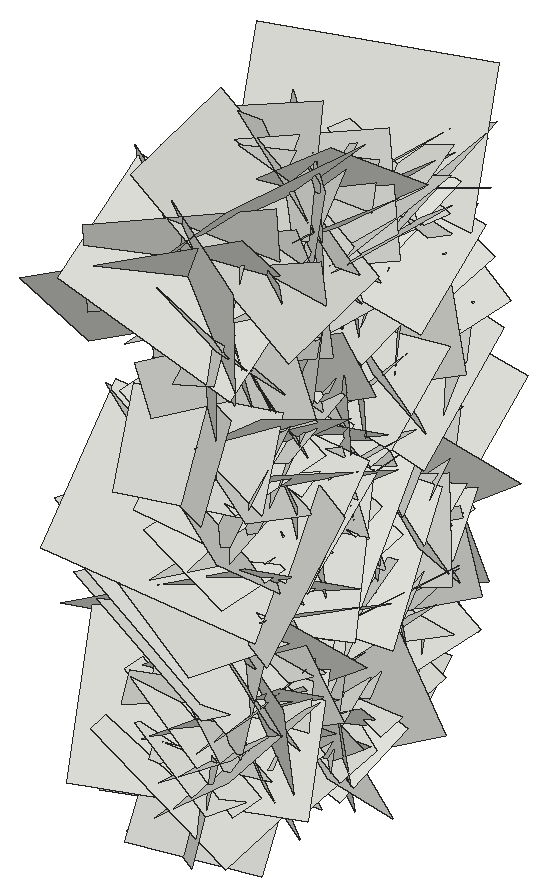
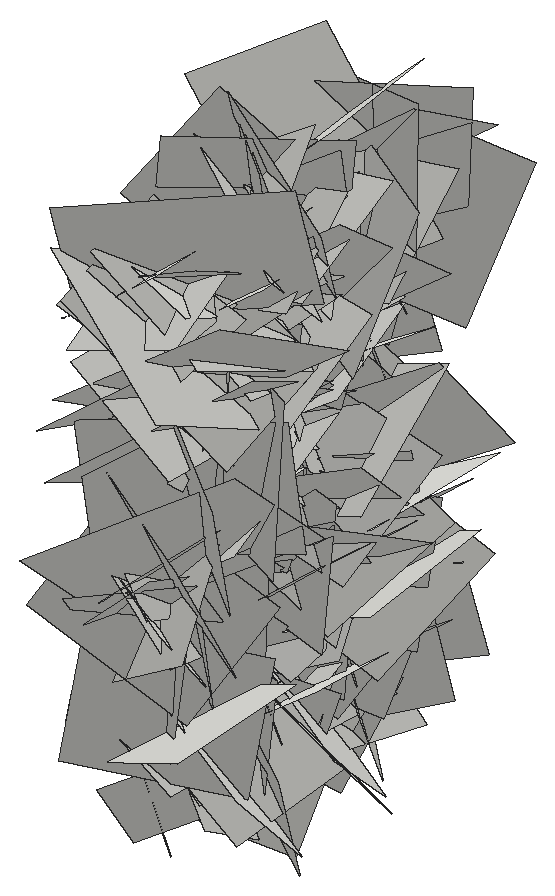
# SketchUp Ruby script. Lengths in inches.
U = 1.inch
M = Sketchup.active_model
def pt(a) = Geom::Point3d.new(a.map { |v| v * U })
def face(e, loops, mat)
  f = e.add_face(loops[0].map { |a| pt(a) })
  loops[1..].each { |l| e.add_face(l.map { |a| pt(a) }).erase! }
  f.material = f.back_material = mat if mat
  f
end
# faces: each face lists its corners as indices into pts; further lists are holes
def faces(e, pts, list, mat = nil) = list.each { |f| face(e, (f[0].is_a?(Array) ? f : [f]).map { |l| l.map { |i| pts[i] } }, mat) }
# xy, xz, yz: faces in a plane at the given z, y or x. An outline is a flat list of corners, or four numbers for a rectangle; further outlines are holes
def ring(l) = l.size == 4 ? [[l[0], l[1]], [l[2], l[1]], [l[2], l[3]], [l[0], l[3]]] : l.each_slice(2).to_a
def flat(e, list, mat, &to3) = list.each { |f| face(e, (f[0].is_a?(Array) ? f : [f]).map { |l| ring(l).map { |u, v| to3.(u, v) } }, mat) }
def xy(e, z, list, mat = nil) = flat(e, list, mat) { |x, y| [x, y, z] }
def xz(e, y, list, mat = nil) = flat(e, list, mat) { |x, z| [x, y, z] }
def yz(e, x, list, mat = nil) = flat(e, list, mat) { |y, z| [x, y, z] }
def lines(e, pts, list) = list.each { |a, b| e.add_line(pt(pts[a]), pt(pts[b])) }
# prism: a flat outline (further loops are holes) pulled along v
def prism(e, loops, v, mat = nil)
  f = face(e, loops, mat); d = Geom::Vector3d.new(v.map { |x| x * U })
  f.pushpull(f.normal.samedirection?(d) ? d.length : -d.length)
end
def box(e, o, s, mat = nil) = prism(e, [[o, [o[0] + s[0], o[1], o[2]], [o[0] + s[0], o[1] + s[1], o[2]], [o[0], o[1] + s[1], o[2]]]], [0, 0, s[2]], mat)
def at(x, y, z, deg = 0) = Geom::Transformation.translation(pt([x, y, z])) * Geom::Transformation.rotation(ORIGIN, Z_AXIS, deg.degrees)
def axes(o, x, y, z) = Geom::Transformation.new([*x, 0, *y, 0, *z, 0, *pt(o).to_a, 1])
def part(name) = M.definitions.add(name)
# library, detail: a bought-in or finely detailed component or shape, given as its bounding box
def library(name, o, s) = part(name).tap { |d| box(d.entities, o, s) }
def detail(e, o, s) = box(e.add_group.entities, o, s)
def put(e, d, t, mat = nil) = e.add_instance(d, t).tap { |i| i.material = mat if mat }
def group(e, t, mat = nil) = e.add_group.tap { |g| g.transformation = t; g.material = mat if mat }.entities
root = M.entities
c1 = part("Component\#6")
p = [[0.01,0,0],[0,3.24,4.54],[4.32,3.24,4.54],[4.33,0,0]]
faces(c1.entities,p,[[0,1,2,3]])
put(root,c1,axes([18.5,182.27,16.13],[-0.23771,-0.47409,1.27281],[-0.00404,1.29026,0.47991],[-1.43973,0.07465,-0.2115]))
put(root,c1,axes([18.5,189.11,8.53],[-0.25892,-1.11224,-0.53402],[-0.14932,-0.51568,1.13849],[-1.29927,0.28091,-0.02442]))
put(root,c1,axes([18.5,193.85,16.74],[-0.30124,-1.14539,-0.57535],[0.00001,-0.58933,1.17321],[-1.35869,0.25394,0.12757]))
put(root,c1,axes([18.5,184.58,6.82],[-0.16596,-1.29847,0.14138],[-0.0614,0.14916,1.30572],[-1.38315,0.14917,-0.07492]))
put(root,c1,axes([18.5,183.54,2.14],[-0.03864,0.84179,0.92004],[-0.33491,0.88417,-0.82148],[-1.27872,-0.257,0.18735]))
put(root,c1,axes([18.5,180.76,23.09],[-0.06995,0.91309,-0.96842],[-0.10566,-0.97028,-0.90805],[-1.4069,0.02747,0.11634]))
put(root,c1,axes([18.5,187.39,3.1875],[-0.10139,0.89849,0.89189],[-0.1671,0.87902,-0.90243],[-1.33152,-0.17873,0.04534]))
put(root,c1,axes([18.5,189.55,17.94],[-0.16397,-1.09761,-0.83604],[0.11999,-0.84854,1.09307],[-1.45761,0.05363,0.18403]))
put(root,c1,axes([18.5,193.03,3.2],[-0.23388,-1.096,0.27231],[-0.13541,0.2999,1.10354],[-1.1894,0.18138,-0.17918]))
put(root,c1,axes([18.5,184.34,4.6],[-0.11485,-1.15497,0.26483],[-0.19184,0.27894,1.14248],[-1.2413,0.06375,-0.20107]))
put(root,c1,axes([18.5,186.39,13.5625],[-0.22643,-0.80881,0.81079],[-0.0736,0.83241,0.81208],[-1.21171,0.10058,-0.20084]))
put(root,c1,axes([18.5,188.34,12.62],[-0.20954,0.481,1.15591],[0.07101,1.17261,-0.47649],[-1.32521,-0.01322,-0.2083]))
put(root,c1,axes([18.5,184,8.18],[0.02134,-1.06466,0.81449],[-0.04088,0.81378,1.06469],[-1.42032,-0.03942,-0.01841]))
put(root,c1,axes([18.5,184.23,21.55],[-0.30098,0.54789,0.85036],[-0.10123,0.86476,-0.58905],[-1.06749,-0.23649,-0.1839]))
put(root,c1,axes([18.5,183.88,15.08],[0.0404,1.11797,-0.62329],[-0.16276,-0.61507,-1.11262],[-1.34698,0.10785,0.11575]))
put(root,c1,axes([18.5,195.54,11.625],[-0.04246,-1.00606,-0.92627],[0.11693,-0.92602,1.00103],[-1.44486,-0.04538,0.10823]))
put(root,c1,axes([18.5,186.02,17.55],[-0.12484,-0.91824,0.67786],[-0.09261,0.68671,0.91505],[-1.20627,0.04231,-0.14041]))
put(root,c1,axes([18.5,185.87,11.99],[-0.00632,-0.88407,-1.06115],[0.10628,-1.05864,0.88141],[-1.46017,-0.07323,0.06874]))
put(root,c1,axes([18.5,192.77,15.58],[-0.03721,-0.16955,-1.17702],[-0.1418,-1.1695,0.17246],[-1.25252,0.13744,0.01545]))
put(root,c1,axes([18.5,186.66,10.07],[0.09303,-0.2424,1.37134],[0.00293,1.37409,0.24271],[-1.47615,-0.01254,0.08691]))
put(root,c1,axes([18.5,182.38,2.76],[-0.16715,0.82367,0.72398],[-0.09449,0.71938,-0.83785],[-1.15857,-0.1775,-0.03612]))
put(root,c1,axes([18.5,185.25,0.97],[-0.15144,0.45294,1.0525],[-0.02813,1.05906,-0.45936],[-1.21425,-0.08102,-0.12063]))
put(root,c1,axes([18.5,184.5,10.44],[-0.20009,0.552,-0.98447],[0.02572,-0.99592,-0.56307],[-1.1961,-0.11375,0.15258]))
put(root,c1,axes([18.5,180.93,10.86],[0.17521,1.15715,-0.62152],[-0.20897,-0.59747,-1.1648],[-1.37654,0.23798,0.09772]))
put(root,c1,axes([18.5,185.31,6.45],[0.03902,-0.20515,1.15818],[-0.22164,1.13915,0.20842],[-1.22693,-0.21231,-0.00082]))
put(root,c1,axes([18.5,183.02,16.38],[0.02893,-0.8566,0.75588],[-0.26219,0.73373,0.84043],[-1.18223,-0.18368,-0.16789]))
put(root,c1,axes([18.5,190.12,11.53],[0.21117,-0.99907,-0.90649],[-0.1512,-0.92678,0.99009],[-1.42194,-0.04983,-0.2399]))
put(root,c1,axes([18.5,188.7,21.97],[-0.14471,1.28216,-0.28655],[0.25359,-0.25902,-1.27293],[-1.36933,-0.18346,-0.20546]))
put(root,c1,axes([18.5,189.36,1.43],[0.09807,-1.35815,-0.14277],[0.05055,-0.1398,1.36078],[-1.44669,-0.09695,0.03787]))
put(root,c1,axes([18.5,194.04,23.84],[0.15699,-0.54259,-1.24113],[-0.03696,-1.24964,0.54215],[-1.43535,-0.02717,-0.14971]))
put(root,c1,axes([18.5,188.23,7.57],[-0.0913,-1.12353,0.75234],[0.27462,0.72618,1.11413],[-1.40673,0.21468,0.16867]))
put(root,c1,axes([18.5,192.17,8.01],[-0.17438,0.53527,-0.89237],[-0.02164,-0.90494,-0.53904],[-1.10282,-0.06688,0.15168]))
put(root,c1,axes([18.5,182.53,23.48],[-0.24403,0.37129,-0.99391],[0.1038,-1.00526,-0.39821],[-1.11985,-0.17408,0.17968]))
put(root,c1,axes([18.5,182.44,13.63],[0.1579,1.28482,-0.45217],[0.02165,-0.45692,-1.2916],[-1.44363,0.13368,-0.06883]))
put(root,c1,axes([18.5,189.08,9.2],[0.13088,0.55221,1.09741],[-0.12619,1.10312,-0.54169],[-1.29609,-0.05164,0.16356]))
put(root,c1,axes([18.5,187.9375,5.11],[-0.04973,-1.23753,-0.07043],[0.13139,-0.07481,1.23194],[-1.30732,0.03956,0.12649]))
put(root,c1,axes([14.53,190.35,18.26],[-0.16101,-0.65287,0.16772],[-0.08445,0.18811,0.66008],[0.7095,-0.12576,0.11663]))
put(root,c1,axes([18.5,186.43,6.6],[0.00451,1.27416,-0.10814],[0.14001,-0.108,-1.26731],[-1.34821,-0.00695,-0.13197]))
put(root,c1,axes([18.5,185.36,5.79],[-0.02078,-1.22604,-0.15411],[0.11589,-0.15525,1.22117],[-1.3047,0.00574,0.11093]))
put(root,c1,axes([18.5,188.68,19.83],[0.08458,1.11358,0.50301],[0.01593,0.50315,-1.11627],[-1.29513,0.07891,0.01912]))
put(root,c1,axes([18.5,186.13,19.34],[-0.13168,0.96657,0.23982],[-0.01085,0.24043,-0.97432],[-1.05558,-0.12304,-0.0199]))
put(root,c1,axes([14.53,191.11,1.26],[-0.04561,-0.57908,-0.31344],[-0.1156,-0.3035,0.57569],[0.68833,-0.08935,0.07592]))
put(root,c1,axes([18.5,187.26,9.21],[-0.06299,-0.71122,-0.64775],[-0.16214,-0.63375,0.70987],[-1.00673,0.14657,-0.0738]))
put(root,c1,axes([18.5,187.48,17.59],[0.04794,-0.78864,0.66349],[-0.19289,0.64758,0.78214],[-1.07529,-0.15133,-0.11072]))
put(root,c1,axes([18.5,180.4,17.125],[0.23878,-0.31981,1.17522],[-0.15258,1.17979,0.34864],[-1.28199,-0.19998,0.17739]))
put(root,c1,axes([18.5,185.11,13.22],[-0.08906,-0.95701,-0.12674],[-0.0585,-0.12225,0.95969],[-1.02162,0.09043,-0.0439]))
put(root,c1,axes([18.5,191.125,9.45],[0.23474,-0.88576,-0.93612],[-0.00151,-0.95001,0.89856],[-1.36608,-0.15116,-0.16185]))
put(root,c1,axes([18.5,184.05,20.67],[-0.10102,0.73684,0.6989],[0.04073,0.70408,-0.73707],[-1.07574,-0.04254,-0.09354]))
put(root,c1,axes([18.5,181.08,20.02],[0.00536,1.00575,0.03656],[-0.10796,0.03689,-1.00058],[-1.06133,0.00133,0.10197]))
put(root,c1,axes([18.5,185.52,6.2],[0.2751,-0.65276,-1.16933],[0.03559,-1.18754,0.67037],[-1.41909,-0.15632,-0.20987]))
put(root,c1,axes([14.53,188.8,6.44],[-0.14743,-0.18272,-0.74199],[-0.06403,-0.74919,0.19581],[0.80747,-0.09277,-0.11994]))
put(root,c1,axes([18.5,179.32,18.3],[-0.15069,0.54422,0.74866],[0.00735,0.75804,-0.54972],[-0.98107,-0.07791,-0.11911]))
put(root,c1,axes([18.5,184.31,4.6],[-0.1576,-0.1516,-1.0147],[0.15202,-1.0183,0.13112],[-1.07684,-0.12157,0.16702]))
put(root,c1,axes([14.53,186.3,8.38],[0.07617,0.47932,0.41871],[-0.13681,0.42359,-0.46276],[0.66062,0.03245,-0.14411]))
put(root,c1,axes([18.5,184.41,20.14],[0.03821,-1.03167,-0.60174],[0.15497,-0.59368,1.0266],[-1.25647,-0.1046,0.10832]))
put(root,c1,axes([18.5,194.3,13.93],[0.22437,-1.23478,-0.60854],[0.19245,-0.58527,1.25072],[-1.44644,-0.26941,0.07201]))
put(root,c1,axes([14.53,187.98,11.49],[-0.12716,0.81746,0.20835],[-0.15,0.18797,-0.81896],[0.88154,0.1499,-0.10929]))
put(root,c1,axes([14.53,186.0625,6.1],[-0.08854,0.52684,0.45627],[0.00383,0.45985,-0.53032],[0.73876,0.06076,0.05744]))
put(root,c1,axes([18.5,181.29,16.68],[-0.08133,-0.245,0.96212],[0.05676,0.96256,0.24939],[-1.05086,0.07095,-0.06099]))
put(root,c1,axes([18.5,184.19,13.53],[-0.08078,-0.49886,0.79857],[-0.01528,0.8017,0.49945],[-0.99796,0.02811,-0.07229]))
put(root,c1,axes([18.5,187.61,11.62],[0.28203,-0.58282,-1.12773],[-0.01249,-1.15332,0.59327],[-1.34554,-0.11146,-0.24188]))
put(root,c1,axes([14.53,183.1,18.89],[-0.1435,0.17311,-0.85276],[-0.14536,-0.85648,-0.1521],[0.91084,-0.10941,-0.15862]))
put(root,c1,axes([14.53,183.83,7.3125],[-0.02805,0.62389,-0.09529],[0.05665,-0.09282,-0.62253],[0.66659,0.03414,0.0489]))
put(root,c1,axes([18.5,184.51,1.15],[0.01173,-1.06899,-0.22188],[0.10644,-0.21996,1.06472],[-1.15237,-0.0312,0.09608]))
put(root,c1,axes([18.5,186.9375,3.03],[-0.11563,0.62873,-0.58509],[-0.05581,-0.59358,-0.62803],[-0.90867,-0.04354,0.11303]))
put(root,c1,axes([14.53,189.45,1.42],[0.1039,0.30381,0.53974],[-0.07033,0.54846,-0.29667],[0.65275,0.01074,-0.11787]))
put(root,c1,axes([14.53,184.54,3.47],[-0.05739,0.5962,-0.42459],[-0.0201,-0.42675,-0.59681],[0.77559,0.03305,-0.04688]))
put(root,c1,axes([18.5,185.64,19.96],[0.2349,1.07139,0.39402],[-0.08081,0.41437,-1.08385],[-1.20734,0.18072,0.1492]))
put(root,c1,axes([18.5,186.72,4.72],[0.08241,-0.91883,0.29273],[-0.13826,0.28096,0.91654],[-1.0128,-0.11312,-0.1013]))
put(root,c1,axes([18.5,190.33,17.67],[-0.17424,0.82504,0.17436],[0.04616,0.18571,-0.83769],[-0.89267,-0.15144,-0.07735]))
put(root,c1,axes([18.5,179.97,24.47],[0.23304,1.36821,0.06434],[0.25904,0.02493,-1.36533],[-1.42861,0.2277,-0.23708]))
put(root,c1,axes([14.53,184.43,15.42],[-0.12844,-0.04329,0.74472],[0.08874,0.74892,0.05716],[0.78574,-0.09166,0.11528]))
put(root,c1,axes([18.5,189.57,16.9],[-0.06471,0.53395,-0.71324],[-0.01751,-0.71546,-0.53421],[-0.94426,-0.02333,0.05878]))
put(root,c1,axes([18.5,191,16.96],[0.17643,-1.14926,-0.11809],[0.05518,-0.11173,1.16072],[-1.22339,-0.17078,0.03532]))
put(root,c1,axes([14.53,186.92,8.78],[-0.10246,-0.30095,0.75916],[-0.04625,0.76527,0.29782],[0.86439,0.00528,0.10592]))
put(root,c1,axes([18.5,180.14,11.99],[0.0212,0.75168,0.8023],[0.17372,0.79143,-0.74558],[-1.15236,0.13314,-0.09764]))
put(root,c1,axes([18.5,185.08,2.16],[-0.06404,-1.02262,-0.11109],[0.17979,-0.11966,1.00929],[-1.07543,0.04089,0.17535]))
put(root,c1,axes([18.5,187.17,12.95],[0.05814,-0.16279,1.09674],[0.14666,1.09051,0.15494],[-1.1661,0.12904,0.07417]))
put(root,c1,axes([18.5,187.85,22.99],[-0.09057,-0.06637,-0.91857],[0.07612,-0.92019,0.05981],[-0.97325,-0.06579,0.09016]))
put(root,c1,axes([14.53,183.375,2.21],[0.01982,-0.33114,-0.74136],[-0.16849,-0.7287,0.32148],[0.84401,-0.13769,0.08159]))
put(root,c1,axes([14.53,192.83,7.86],[0.1126,-0.65912,-0.17655],[-0.1088,-0.19208,0.65534],[0.71507,0.07456,0.12751]))
put(root,c1,axes([18.5,183.46,7.83],[0.1867,0.36795,-0.96583],[-0.13041,-0.96532,-0.39019],[-1.08777,0.17888,-0.11899]))
put(root,c1,axes([18.5,186.63,-0.64],[0.14781,-0.37723,1.01914],[0.01271,1.02797,0.37886],[-1.15185,-0.03706,0.13496]))
put(root,c1,axes([18.5,183.61,1.59],[-0.06331,-0.78644,0.46242],[0.03597,0.46118,0.7887],[-0.96639,0.06869,-0.00094]))
put(root,c1,axes([18.5,185.25,15.47],[-0.04372,0.77316,0.71524],[0.20224,0.70943,-0.75587],[-1.09798,0.09988,-0.16771]))
put(root,c1,axes([18.5,185.13,2.21],[-0.09174,0.69928,0.36],[-0.10121,0.35015,-0.7031],[-0.82753,-0.12035,0.04608]))
put(root,c1,axes([14.53,192.38,19.24],[0.04943,-0.7355,0.057],[-0.07325,0.05251,0.73407],[0.77853,0.05163,0.06545]))
put(root,c1,axes([18.5,181.6,11.88],[-0.05183,0.72565,0.67247],[0.15864,0.67097,-0.71314],[-1.03662,0.0664,-0.14276]))
put(root,c1,axes([14.53,185.26,12.26],[-0.159,0.84642,0.10737],[0.04855,0.11685,-0.85715],[0.9031,0.14274,0.06498]))
put(root,c1,axes([14.53,185.94,13.1875],[-0.12339,0.16979,-0.82402],[0.01755,-0.83125,-0.17361],[0.89164,0.03986,-0.11061]))
put(root,c1,axes([14.53,183.19,13.8],[-0.02762,0.65605,0.3231],[0.06014,0.32414,-0.6536],[0.77284,-0.00178,0.06241]))
put(root,c1,axes([18.5,184.53,11.29],[0.10396,-0.95246,0.37472],[0.04499,0.37989,0.95451],[-1.084,-0.07558,0.07555]))
put(root,c1,axes([18.5,192.08,20.31],[-0.05296,-0.67773,-0.30339],[-0.1724,-0.2867,0.66724],[-0.76797,0.11109,-0.12886]))
put(root,c1,axes([14.53,192.03,8.33],[-0.03388,0.22508,-0.86549],[-0.13142,-0.8588,-0.21876],[0.93879,-0.1121,-0.06186]))
put(root,c1,axes([14.53,185.14,8.49],[0.08576,-0.66072,-0.04627],[0.0456,-0.04128,0.66459],[0.70059,0.08356,-0.03759]))
put(root,c1,axes([14.53,183.28,17.73],[-0.09647,-0.26045,0.74001],[0.11879,0.73302,0.27177],[0.82305,-0.13632,0.04751]))
put(root,c1,axes([14.53,193.37,9.31],[-0.05697,-0.46717,-0.61186],[0.09106,-0.61316,0.46062],[0.81091,0.03603,-0.09471]))
put(root,c1,axes([14.53,191.46,9.82],[-0.08538,-0.06629,-0.92063],[-0.09555,-0.91915,0.07407],[0.97372,-0.09601,-0.07345]))
put(root,c1,axes([14.53,191.35,2.27],[-0.06694,-0.86655,-0.10749],[-0.04783,-0.10439,0.86806],[0.92435,-0.06816,0.03713]))
put(root,c1,axes([14.53,190.84,12.42],[0.00848,-0.77925,-0.15089],[-0.03038,-0.15108,0.77873],[0.8408,0.0024,0.02966]))
put(root,c1,axes([14.53,182.98,9.92],[0.09782,-0.62966,-0.10425],[0.08997,-0.09229,0.63256],[0.67052,0.10424,-0.06967]))
put(root,c1,axes([14.53,180.19,4.07],[0.08532,0.68038,-0.07405],[0.04058,-0.07892,-0.68351],[0.72433,-0.07573,0.04702]))
put(root,c1,axes([14.53,183.91,5.17],[-0.1157,0.58195,-0.7538],[-0.08085,-0.76164,-0.57696],[1.0062,0.00571,-0.13304]))
put(root,c1,axes([14.53,182.875,15.8],[-0.04284,-0.30855,-0.78276],[-0.017,-0.78324,0.30957],[0.8917,-0.02976,-0.0317]))
put(root,c1,axes([18.5,184.33,2.33],[0.23495,-0.78095,0.69461],[-0.033,0.70481,0.80235],[-1.10738,-0.18669,0.12346]))
put(root,c1,axes([18.5,189.86,21.06],[0.09411,0.75469,-0.30292],[-0.23058,-0.27158,-0.74036],[-0.83059,0.16091,0.17121]))
put(root,c1,axes([18.5,189.65,5.54],[-0.06955,0.77959,0.08211],[-0.00823,0.08175,-0.78235],[-0.8309,-0.06607,0.00087]))
put(root,c1,axes([18.5,192.04,5.47],[0.24252,-0.79203,0.72828],[0.0092,0.7459,0.80846],[-1.14049,-0.1624,0.16139]))
put(root,c1,axes([18.5,184.16,21.8125],[0.07155,0.99261,-0.10082],[0.11355,-0.10768,-0.9884],[-1.05147,0.05592,-0.1136]))
put(root,c1,axes([14.53,184.68,7.1],[-0.07537,-0.21143,-0.85755],[-0.01444,-0.85996,0.21315],[0.93612,-0.03029,-0.06575]))
put(root,c1,axes([14.53,187.95,18.35],[-0.24952,-0.85217,0.60628],[-0.01294,0.62364,0.87183],[1.1085,-0.18454,0.14665]))
put(root,c1,axes([18.5,188.38,23.95],[0.14683,-0.05211,-1.06804],[0.1506,-1.06652,0.07046],[-1.12342,-0.14978,-0.13015]))
put(root,c1,axes([14.53,188.38,23.95],[-0.14683,-0.05211,-1.06804],[-0.1506,-1.06652,0.07046],[1.12342,-0.14978,-0.13015]))
put(root,c1,axes([18.5,187.95,18.35],[0.24952,-0.85217,0.60628],[0.01294,0.62364,0.87183],[-1.1085,-0.18454,0.14665]))
put(root,c1,axes([18.5,184.68,7.1],[0.07537,-0.21143,-0.85755],[0.01444,-0.85996,0.21315],[-0.93612,-0.03029,-0.06575]))
put(root,c1,axes([14.53,184.16,21.8125],[-0.07155,0.99261,-0.10082],[-0.11355,-0.10768,-0.9884],[1.05147,0.05592,-0.1136]))
put(root,c1,axes([14.53,192.04,5.47],[-0.24252,-0.79203,0.72828],[-0.0092,0.7459,0.80846],[1.14049,-0.1624,0.16139]))
put(root,c1,axes([14.53,189.65,5.54],[0.06955,0.77959,0.08211],[0.00823,0.08175,-0.78235],[0.8309,-0.06607,0.00087]))
put(root,c1,axes([14.53,189.86,21.06],[-0.09411,0.75469,-0.30292],[0.23058,-0.27158,-0.74036],[0.83059,0.16091,0.17121]))
put(root,c1,axes([14.53,184.33,2.33],[-0.23495,-0.78095,0.69461],[0.033,0.70481,0.80235],[1.10738,-0.18669,0.12346]))
put(root,c1,axes([18.5,182.875,15.8],[0.04284,-0.30855,-0.78276],[0.017,-0.78324,0.30957],[-0.8917,-0.02976,-0.0317]))
put(root,c1,axes([18.5,183.91,5.17],[0.1157,0.58195,-0.7538],[0.08085,-0.76164,-0.57696],[-1.0062,0.00571,-0.13304]))
put(root,c1,axes([18.5,180.19,4.07],[-0.08532,0.68038,-0.07405],[-0.04058,-0.07892,-0.68351],[-0.72433,-0.07573,0.04702]))
put(root,c1,axes([18.5,182.98,9.92],[-0.09782,-0.62966,-0.10425],[-0.08997,-0.09229,0.63256],[-0.67052,0.10424,-0.06967]))
put(root,c1,axes([18.5,190.84,12.42],[-0.00848,-0.77925,-0.15089],[0.03038,-0.15108,0.77873],[-0.8408,0.0024,0.02966]))
put(root,c1,axes([18.5,191.35,2.27],[0.06694,-0.86655,-0.10749],[0.04783,-0.10439,0.86806],[-0.92435,-0.06816,0.03713]))
put(root,c1,axes([18.5,191.46,9.82],[0.08538,-0.06629,-0.92063],[0.09555,-0.91915,0.07407],[-0.97372,-0.09601,-0.07345]))
put(root,c1,axes([18.5,193.37,9.31],[0.05697,-0.46717,-0.61186],[-0.09106,-0.61316,0.46062],[-0.81091,0.03603,-0.09471]))
put(root,c1,axes([18.5,183.28,17.73],[0.09647,-0.26045,0.74001],[-0.11879,0.73302,0.27177],[-0.82305,-0.13632,0.04751]))
put(root,c1,axes([18.5,185.14,8.49],[-0.08576,-0.66072,-0.04627],[-0.0456,-0.04128,0.66459],[-0.70059,0.08356,-0.03759]))
put(root,c1,axes([18.5,192.03,8.33],[0.03388,0.22508,-0.86549],[0.13142,-0.8588,-0.21876],[-0.93879,-0.1121,-0.06186]))
put(root,c1,axes([14.53,192.08,20.31],[0.05296,-0.67773,-0.30339],[0.1724,-0.2867,0.66724],[0.76797,0.11109,-0.12886]))
put(root,c1,axes([14.53,184.53,11.29],[-0.10396,-0.95246,0.37472],[-0.04499,0.37989,0.95451],[1.084,-0.07558,0.07555]))
put(root,c1,axes([18.5,183.19,13.8],[0.02762,0.65605,0.3231],[-0.06014,0.32414,-0.6536],[-0.77284,-0.00178,0.06241]))
put(root,c1,axes([18.5,185.94,13.1875],[0.12339,0.16979,-0.82402],[-0.01755,-0.83125,-0.17361],[-0.89164,0.03986,-0.11061]))
put(root,c1,axes([18.5,185.26,12.26],[0.159,0.84642,0.10737],[-0.04855,0.11685,-0.85715],[-0.9031,0.14274,0.06498]))
put(root,c1,axes([14.53,181.6,11.88],[0.05183,0.72565,0.67247],[-0.15864,0.67097,-0.71314],[1.03662,0.0664,-0.14276]))
put(root,c1,axes([18.5,192.38,19.24],[-0.04943,-0.7355,0.057],[0.07325,0.05251,0.73407],[-0.77853,0.05163,0.06545]))
put(root,c1,axes([14.53,185.13,2.21],[0.09174,0.69928,0.36],[0.10121,0.35015,-0.7031],[0.82753,-0.12035,0.04608]))
put(root,c1,axes([14.53,185.25,15.47],[0.04372,0.77316,0.71524],[-0.20224,0.70943,-0.75587],[1.09798,0.09988,-0.16771]))
put(root,c1,axes([14.53,183.61,1.59],[0.06331,-0.78644,0.46242],[-0.03597,0.46118,0.7887],[0.96639,0.06869,-0.00094]))
put(root,c1,axes([14.53,186.63,-0.64],[-0.14781,-0.37723,1.01914],[-0.01271,1.02797,0.37886],[1.15185,-0.03706,0.13496]))
put(root,c1,axes([14.53,183.46,7.83],[-0.1867,0.36795,-0.96583],[0.13041,-0.96532,-0.39019],[1.08777,0.17888,-0.11899]))
put(root,c1,axes([18.5,192.83,7.86],[-0.1126,-0.65912,-0.17655],[0.1088,-0.19208,0.65534],[-0.71507,0.07456,0.12751]))
put(root,c1,axes([18.5,183.375,2.21],[-0.01982,-0.33114,-0.74136],[0.16849,-0.7287,0.32148],[-0.84401,-0.13769,0.08159]))
put(root,c1,axes([14.53,187.85,22.99],[0.09057,-0.06637,-0.91857],[-0.07612,-0.92019,0.05981],[0.97325,-0.06579,0.09016]))
put(root,c1,axes([14.53,187.17,12.95],[-0.05814,-0.16279,1.09674],[-0.14666,1.09051,0.15494],[1.1661,0.12904,0.07417]))
put(root,c1,axes([14.53,185.08,2.16],[0.06404,-1.02262,-0.11109],[-0.17979,-0.11966,1.00929],[1.07543,0.04089,0.17535]))
put(root,c1,axes([14.53,180.14,11.99],[-0.0212,0.75168,0.8023],[-0.17372,0.79143,-0.74558],[1.15236,0.13314,-0.09764]))
put(root,c1,axes([18.5,186.92,8.78],[0.10246,-0.30095,0.75916],[0.04625,0.76527,0.29782],[-0.86439,0.00528,0.10592]))
put(root,c1,axes([14.53,191,16.96],[-0.17643,-1.14926,-0.11809],[-0.05518,-0.11173,1.16072],[1.22339,-0.17078,0.03532]))
put(root,c1,axes([14.53,189.57,16.9],[0.06471,0.53395,-0.71324],[0.01751,-0.71546,-0.53421],[0.94426,-0.02333,0.05878]))
put(root,c1,axes([18.5,184.43,15.42],[0.12844,-0.04329,0.74472],[-0.08874,0.74892,0.05716],[-0.78574,-0.09166,0.11528]))
put(root,c1,axes([14.53,179.97,24.47],[-0.23304,1.36821,0.06434],[-0.25904,0.02493,-1.36533],[1.42861,0.2277,-0.23708]))
put(root,c1,axes([14.53,190.33,17.67],[0.17424,0.82504,0.17436],[-0.04616,0.18571,-0.83769],[0.89267,-0.15144,-0.07735]))
put(root,c1,axes([14.53,186.72,4.72],[-0.08241,-0.91883,0.29273],[0.13826,0.28096,0.91654],[1.0128,-0.11312,-0.1013]))
put(root,c1,axes([14.53,185.64,19.96],[-0.2349,1.07139,0.39402],[0.08081,0.41437,-1.08385],[1.20734,0.18072,0.1492]))
put(root,c1,axes([18.5,184.54,3.47],[0.05739,0.5962,-0.42459],[0.0201,-0.42675,-0.59681],[-0.77559,0.03305,-0.04688]))
put(root,c1,axes([18.5,189.45,1.42],[-0.1039,0.30381,0.53974],[0.07033,0.54846,-0.29667],[-0.65275,0.01074,-0.11787]))
put(root,c1,axes([14.53,186.9375,3.03],[0.11563,0.62873,-0.58509],[0.05581,-0.59358,-0.62803],[0.90867,-0.04354,0.11303]))
put(root,c1,axes([14.53,184.51,1.15],[-0.01173,-1.06899,-0.22188],[-0.10644,-0.21996,1.06472],[1.15237,-0.0312,0.09608]))
put(root,c1,axes([18.5,183.83,7.3125],[0.02805,0.62389,-0.09529],[-0.05665,-0.09282,-0.62253],[-0.66659,0.03414,0.0489]))
put(root,c1,axes([18.5,183.1,18.89],[0.1435,0.17311,-0.85276],[0.14536,-0.85648,-0.1521],[-0.91084,-0.10941,-0.15862]))
put(root,c1,axes([14.53,187.61,11.62],[-0.28203,-0.58282,-1.12773],[0.01249,-1.15332,0.59327],[1.34554,-0.11146,-0.24188]))
put(root,c1,axes([14.53,184.19,13.53],[0.08078,-0.49886,0.79857],[0.01528,0.8017,0.49945],[0.99796,0.02811,-0.07229]))
put(root,c1,axes([14.53,181.29,16.68],[0.08133,-0.245,0.96212],[-0.05676,0.96256,0.24939],[1.05086,0.07095,-0.06099]))
put(root,c1,axes([18.5,186.0625,6.1],[0.08854,0.52684,0.45627],[-0.00383,0.45985,-0.53032],[-0.73876,0.06076,0.05744]))
put(root,c1,axes([18.5,187.98,11.49],[0.12716,0.81746,0.20835],[0.15,0.18797,-0.81896],[-0.88154,0.1499,-0.10929]))
